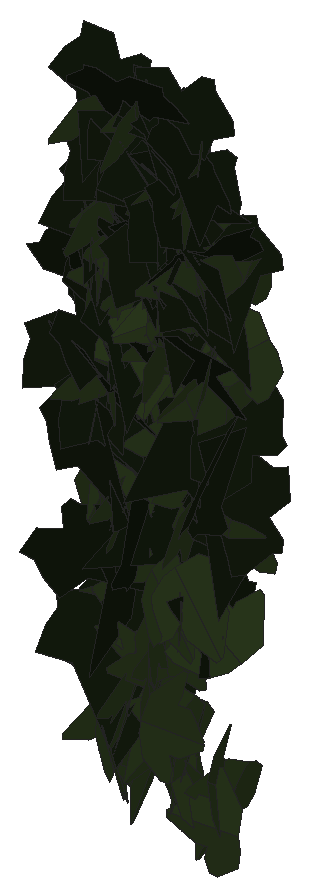
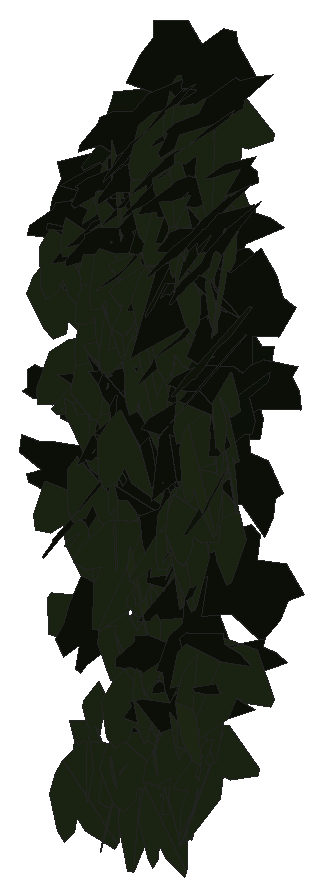
# SketchUp Ruby script. Lengths in inches.
U = 1.inch
M = Sketchup.active_model
def pt(a) = Geom::Point3d.new(a.map { |v| v * U })
def face(e, loops, mat)
  f = e.add_face(loops[0].map { |a| pt(a) })
  loops[1..].each { |l| e.add_face(l.map { |a| pt(a) }).erase! }
  f.material = f.back_material = mat if mat
  f
end
# faces: each face lists its corners as indices into pts; further lists are holes
def faces(e, pts, list, mat = nil) = list.each { |f| face(e, (f[0].is_a?(Array) ? f : [f]).map { |l| l.map { |i| pts[i] } }, mat) }
# xy, xz, yz: faces in a plane at the given z, y or x. An outline is a flat list of corners, or four numbers for a rectangle; further outlines are holes
def ring(l) = l.size == 4 ? [[l[0], l[1]], [l[2], l[1]], [l[2], l[3]], [l[0], l[3]]] : l.each_slice(2).to_a
def flat(e, list, mat, &to3) = list.each { |f| face(e, (f[0].is_a?(Array) ? f : [f]).map { |l| ring(l).map { |u, v| to3.(u, v) } }, mat) }
def xy(e, z, list, mat = nil) = flat(e, list, mat) { |x, y| [x, y, z] }
def xz(e, y, list, mat = nil) = flat(e, list, mat) { |x, z| [x, y, z] }
def yz(e, x, list, mat = nil) = flat(e, list, mat) { |y, z| [x, y, z] }
def lines(e, pts, list) = list.each { |a, b| e.add_line(pt(pts[a]), pt(pts[b])) }
# prism: a flat outline (further loops are holes) pulled along v
def prism(e, loops, v, mat = nil)
  f = face(e, loops, mat); d = Geom::Vector3d.new(v.map { |x| x * U })
  f.pushpull(f.normal.samedirection?(d) ? d.length : -d.length)
end
def box(e, o, s, mat = nil) = prism(e, [[o, [o[0] + s[0], o[1], o[2]], [o[0] + s[0], o[1] + s[1], o[2]], [o[0], o[1] + s[1], o[2]]]], [0, 0, s[2]], mat)
def at(x, y, z, deg = 0) = Geom::Transformation.translation(pt([x, y, z])) * Geom::Transformation.rotation(ORIGIN, Z_AXIS, deg.degrees)
def axes(o, x, y, z) = Geom::Transformation.new([*x, 0, *y, 0, *z, 0, *pt(o).to_a, 1])
def part(name) = M.definitions.add(name)
# library, detail: a bought-in or finely detailed component or shape, given as its bounding box
def library(name, o, s) = part(name).tap { |d| box(d.entities, o, s) }
def detail(e, o, s) = box(e.add_group.entities, o, s)
def put(e, d, t, mat = nil) = e.add_instance(d, t).tap { |i| i.material = mat if mat }
def group(e, t, mat = nil) = e.add_group.tap { |g| g.transformation = t; g.material = mat if mat }.entities
root = M.entities
M.materials.add("efeu1").color = [18, 25, 13]
M.materials.add("efeu2").color = [43, 57, 29]
c1 = part("ivyleaf_9")
p = [[1.54,2.16,1.25],[1.36,2.04,1.19],[-0.21,0.99,0.68],[-0.71,1.11,0.82],[-0.85,0.86,0.67],[-0.8,0.17,0.21],
  [-0.9,-0.01,0.1],[-0.67,-0.16,-0.02],[-0.08,-0.08,-0.05],[-0.03,-0.6,-0.4],[0.65,-0.88,-0.66],[0.83,-0.6,-0.49],
  [1.29,-0.42,-0.43],[1.8125,-0.07,-0.26],[1.21,0.44,0.15]]
faces(c1.entities,p,[[0,1,2,3,4,5,6,7,8,9,10,11,12,13,14]],"efeu1")
c2 = part("ivyleaf_10")
p = [[0,0.5,-0.03],[-0.0625,2.02,-0.43],[-0.19,2.01,-0.46],[-0.54,1.05,-0.29],[-0.52,0.625,-0.18],[-0.83,0.76,-0.28],
  [-1.16,0.64,-0.33],[-1.15,0.33,-0.24],[-0.77,-0.39,0.02],[-0.3,-0.51,0.16],[0.04,-0.48,0.23],[-0.02,2.01,-0.4375],
  [-0.06,2.01,-0.43],[0.04,-0.49,0.23],[0.67,-0.49,0.14],[1.38,0.36,-0.2],[1.375,0.51,-0.24],[0.81,0.65,-0.19],
  [0.62,0.59,-0.15],[0.6,1.09,-0.28],[0.5,1.23,-0.31]]
faces(c2.entities,p,[[0,1,2,3,4,5,6,7,8,9,10],[11,12,0,13,14,15,16,17,18,19,20]],"efeu2")
put(root,c1,axes([21.54,224.6,221.31],[-0.03751,-0.43289,0.24739],[-0.01562,-0.24695,-0.43448],[0.49835,-0.04032,0.005]))
put(root,c2,axes([21.63,224.2,216.18],[-0.33905,-0.31869,-0.18299],[0.15039,0.10685,-0.46472],[0.33531,-0.37017,0.02341]))
put(root,c2,axes([21.72,224,219.07],[0.31446,-0.36783,-0.12576],[-0.0441,0.12696,-0.4816],[0.38623,0.31398,0.0474]))
put(root,c1,axes([21.52,224,219.68],[-0.1222,-0.35359,-0.33173],[0.1348,0.30383,-0.37352],[0.46572,-0.18072,0.02107]))
put(root,c2,axes([21.77,223.86,221.06],[0.21838,-0.23586,-0.38299],[-0.07654,0.40004,-0.29001],[0.44323,0.1853,0.13862]))
put(root,c1,axes([21.34,224.08,220.3],[0.07088,-0.10152,0.48443],[0.46593,-0.15142,-0.0999],[0.16699,0.46558,0.07314]))
put(root,c2,axes([21.79,224.38,218.84],[0.0993,-0.48986,0.01339],[0.00243,-0.01317,-0.49982],[0.49003,0.09933,-0.00023]))
put(root,c2,axes([21.8,224.03,222.69],[-0.16464,-0.46488,-0.08234],[0.03056,0.07653,-0.49316],[0.47113,-0.16742,0.00321]))
put(root,c1,axes([21.51,224.42,220.18],[0.11841,-0.44827,0.18717],[0.08554,-0.1704,-0.46222],[0.47819,0.14148,0.03633]))
put(root,c1,axes([21.47,223.92,218.66],[-0.11306,-0.0302,-0.48611],[0.45319,0.17629,-0.11635],[0.17842,-0.46692,-0.01249]))
put(root,c1,axes([21.7,224.43,223],[-0.10796,-0.47713,0.10338],[-0.03629,-0.09774,-0.48901],[0.48685,-0.11309,-0.01353]))
put(root,c1,axes([21.63,224.67,221.66],[0.00983,-0.48341,0.12736],[0.02799,-0.12665,-0.48288],[0.49912,0.01662,0.02458]))
put(root,c1,axes([21.64,223.83,219.95],[0.31733,-0.28414,-0.26185],[-0.114,0.25491,-0.41476],[0.36919,0.32294,0.097]))
put(root,c2,axes([21.68,224.67,215.83],[0.13204,-0.24449,0.41568],[0.22976,-0.34703,-0.27709],[0.424,0.26419,0.02071]))
put(root,c1,axes([21.55,223.73,217.23],[-0.00624,-0.00511,-0.49993],[0.22683,0.44553,-0.00739],[0.44554,-0.22689,-0.00324]))
put(root,c2,axes([21.8125,224.49,218.18],[-0.0502,-0.33029,0.37201],[0.10917,-0.3721,-0.31564],[0.48535,0.04953,0.10947]))
put(root,c2,axes([21.9,223.93,219.46],[0.37281,-0.24376,-0.22714],[-0.08833,0.25636,-0.42009],[0.32127,0.35335,0.14809]))
put(root,c2,axes([21.625,224.31,220.9],[0.05659,-0.18533,0.46092],[0.33646,-0.32701,-0.1728],[0.3655,0.32972,0.08771]))
put(root,c2,axes([21.93,223.99,219.31],[-0.14495,-0.47492,0.05866],[-0.00922,-0.05851,-0.49648],[0.47844,-0.14501,0.0082]))
put(root,c1,axes([21.79,224.23,221.43],[-0.16768,-0.46006,-0.10113],[0.02624,0.09806,-0.48959],[0.47031,-0.1695,-0.00874]))
put(root,c1,axes([21.49,223.93,219.375],[0.3497,-0.23984,0.26493],[0.21704,-0.15194,-0.42403],[0.28391,0.41157,-0.00216]))
put(root,c2,axes([21.95,224.22,220.9],[0.07397,-0.42517,0.2525],[0.03707,-0.24982,-0.43153],[0.49311,0.08256,-0.00544]))
put(root,c1,axes([21.81,224.09,216.07],[-0.12914,-0.46255,-0.13917],[0.06065,0.12739,-0.47968],[0.47921,-0.14077,0.02321]))
put(root,c2,axes([21.96,223.97,214.81],[-0.14407,0.44926,0.16557],[-0.05725,0.15549,-0.47174],[-0.47536,-0.15489,0.00664]))
put(root,c2,axes([22.04,224.08,214.9375],[-0.31179,-0.38522,-0.06628],[0.04263,0.05077,-0.49559],[0.38855,-0.31468,0.00118]))
put(root,c1,axes([21.81,224.27,222.05],[0.02579,-0.4565,-0.20234],[0.05076,0.20396,-0.45368],[0.49675,0.00286,0.05686]))
put(root,c2,axes([22.09,224.19,221.47],[-0.22555,-0.44544,0.02654],[-0.00874,-0.02533,-0.49928],[0.44615,-0.22569,0.00364]))
put(root,c2,axes([22.05,223.81,221.57],[-0.10457,-0.43547,-0.22234],[0.04754,0.21723,-0.44783],[0.48663,-0.1148,-0.00402]))
put(root,c2,axes([22.24,224.1,215.78],[-0.41311,-0.1799,0.21673],[-0.18645,-0.11371,-0.44978],[0.21112,-0.45244,0.02686]))
put(root,c1,axes([21.92,224.44,216.65],[-0.01109,0.03453,-0.49868],[0.34864,-0.35693,-0.03247],[-0.35823,-0.34844,-0.01616]))
put(root,c1,axes([21.92,223.89,220.99],[0.3725,0.32266,0.08447],[0.06716,0.05147,-0.49279],[-0.3267,0.37847,-0.00499]))
put(root,c2,axes([22.1,224.27,217.8125],[-0.00332,-0.49995,-0.00604],[-0.00328,0.00607,-0.49995],[0.49998,-0.00328,-0.00332]))
put(root,c2,axes([21.79,223.98,217.82],[-0.2951,0.06426,-0.39848],[0.36441,-0.16984,-0.29726],[-0.17356,-0.46586,0.05341]))
put(root,c1,axes([21.89,224.03,219.14],[-0.00986,-0.35825,-0.34865],[0.03018,0.34766,-0.35808],[0.49899,-0.0281,0.01477]))
put(root,c1,axes([21.89,224.51,217.83],[-0.04094,-0.3273,0.37576],[0.07751,-0.37662,-0.31961],[0.49226,0.03209,0.08158]))
put(root,c1,axes([22.02,224.5,216.36],[-0.28969,-0.36336,-0.18453],[0.11155,0.14706,-0.46468],[0.39196,-0.3104,-0.00414]))
put(root,c2,axes([22.18,223.72,214.77],[-0.28123,0.36369,0.19656],[-0.14105,0.13906,-0.45909],[-0.3886,-0.31368,0.02438]))
put(root,c1,axes([22.07,224.48,215.63],[-0.28134,-0.40318,-0.0911],[0.05035,0.07595,-0.49163],[0.41026,-0.2858,-0.00214]))
put(root,c2,axes([22.17,224.39,222.57],[-0.16099,-0.47292,-0.02075],[0.00312,0.02086,-0.49956],[0.47336,-0.16097,-0.00376]))
put(root,c2,axes([22.27,224,220.66],[-0.32795,-0.33807,0.16781],[-0.09723,-0.13913,-0.47031],[0.36469,-0.3411,0.02551]))
put(root,c1,axes([21.93,224.38,222.47],[0.12725,-0.47335,-0.09874],[0.01766,0.10659,-0.48819],[0.48321,0.12075,0.04385]))
put(root,c2,axes([22.18,224.58,214.41],[0.10136,-0.45178,0.18875],[0.0609,-0.17962,-0.46263],[0.48582,0.11678,0.01862]))
put(root,c1,axes([22.28,223.71,223.26],[0.31921,0.28674,-0.25668],[-0.24316,-0.10821,-0.42328],[-0.2983,0.39505,0.07037]))
put(root,c2,axes([22.24,224.1,217.77],[0.11368,-0.46054,-0.15806],[-0.01495,0.15893,-0.47383],[0.48668,0.11246,0.02236]))
put(root,c2,axes([22.21,224.28,220.26],[0.02248,-0.4227,0.26612],[0.06095,-0.26208,-0.42143],[0.49576,0.05138,0.03975]))
put(root,c2,axes([22.25,224.01,215.43],[0.12561,-0.47649,0.08473],[0.03266,-0.079,-0.49264],[0.48286,0.12929,0.01128]))
put(root,c1,axes([22.22,224.21,220.71],[-0.40392,-0.1745,-0.23749],[0.22624,0.0746,-0.4396],[0.18885,-0.46259,0.01869]))
put(root,c2,axes([22.18,224.33,217.67],[-0.05004,0.49059,-0.08256],[0.01801,-0.08114,-0.49304],[-0.49716,-0.05232,-0.00956]))
put(root,c2,axes([22.3,223.96,222.75],[0.06157,-0.4591,-0.18825],[0.01634,0.19147,-0.4616],[0.49593,0.05069,0.03858]))
put(root,c1,axes([22.13,224.23,220.02],[0.01699,-0.48369,0.12551],[0.00108,-0.12555,-0.48398],[0.49971,0.01672,-0.00323]))
put(root,c2,axes([22.34,224.33,220.64],[-0.04908,-0.42906,0.25199],[0.02819,-0.2552,-0.42904],[0.49679,-0.02791,0.04924]))
put(root,c1,axes([22.07,224.22,220.99],[0.13399,-0.39431,0.2767],[0.13414,-0.2453,-0.41453],[0.46266,0.18532,0.04005]))
put(root,c2,axes([22.46,224.5625,215.73],[-0.20626,-0.36949,0.26633],[-0.02981,-0.28079,-0.41264],[0.4545,-0.1861,0.0938]))
put(root,c1,axes([22.2,224.23,222.04],[0.11358,-0.48043,-0.07928],[-0.00004,0.0814,-0.49333],[0.48693,0.11207,0.01845]))
put(root,c2,axes([22.61,224,214.92],[-0.04334,0.0762,-0.49226],[-0.19014,0.45417,0.08705],[0.4604,0.19474,-0.01039]))
put(root,c2,axes([22.58,224.5,214.92],[-0.11121,-0.35561,0.33343],[-0.08608,-0.3223,-0.37244],[0.47982,-0.14024,0.01046]))
put(root,c2,axes([22.44,224.39,215.75],[0.12072,-0.45566,0.16672],[0.07158,-0.1532,-0.47054],[0.4799,0.13748,0.02825]))
put(root,c1,axes([22.38,224.03,217.11],[0.09256,0.2493,0.42342],[-0.14507,-0.3978,0.26592],[0.46946,-0.17208,-0.00131]))
put(root,c1,axes([22.21,224.41,220.78],[0.02091,-0.31296,0.38938],[0.18516,-0.35711,-0.29696],[0.46398,0.15662,0.10096]))
put(root,c1,axes([22.3,224.6,222.65],[0.06585,-0.48486,0.10284],[0.00673,-0.10286,-0.48926],[0.4956,0.06582,-0.00702]))
put(root,c1,axes([22.36,224.57,222.28],[-0.02633,-0.49762,0.04098],[-0.01268,-0.04036,-0.49821],[0.49915,-0.02728,-0.0105]))
put(root,c2,axes([22.57,224.22,221.76],[0.08333,-0.45133,0.19838],[0.02595,-0.1969,-0.45886],[0.49232,0.08677,-0.00939]))
put(root,c2,axes([22.59,224.32,219.61],[0.08317,-0.49286,0.01312],[0.0011,-0.01312,-0.49983],[0.49303,0.08317,-0.0011]))
put(root,c1,axes([22.21,224.35,221.67],[0.22292,-0.30335,0.32907],[0.19664,-0.26386,-0.37644],[0.40204,0.29725,0.00167]))
put(root,c1,axes([22.88,223.66,221.05],[-0.03501,0.07217,0.49352],[-0.24708,0.42726,-0.08001],[-0.43327,-0.24949,0.00575]))
put(root,c1,axes([22.25,223.9,221.87],[0.12975,0.09374,-0.47369],[0.25659,0.40212,0.14986],[0.40906,-0.28198,0.05624]))
put(root,c2,axes([22.74,224.23,214.4],[-0.46927,0.12236,0.12173],[-0.11844,0.02824,-0.48495],[-0.12555,-0.48397,0.00248]))
put(root,c1,axes([22.5,224.57,222.8],[-0.08465,-0.48673,-0.07697],[0.00685,0.07693,-0.494],[0.49273,-0.08469,-0.00635]))
put(root,c2,axes([22.66,224.13,215.75],[-0.3068,-0.37979,-0.10783],[-0.06748,-0.08411,0.48823],[-0.389,0.31414,0.00035]))
put(root,c2,axes([22.53,223.91,220.07],[0.47802,0.14225,0.03556],[0.03133,0.01937,-0.49864],[-0.14324,0.47895,0.00961]))
put(root,c2,axes([22.74,224.25,219.99],[-0.14689,-0.47623,0.04032],[-0.01078,-0.03887,-0.49837],[0.47781,-0.14729,0.00116]))
put(root,c1,axes([22.57,224.2,222.12],[-0.09462,-0.48912,-0.04255],[0.00434,0.0425,-0.49817],[0.49095,-0.09464,-0.0038]))
put(root,c2,axes([22.83,223.77,216.42],[-0.09102,0.37385,0.3193],[-0.24065,0.24929,-0.36047],[-0.42872,-0.2193,0.13455]))
put(root,c2,axes([22.71,224.03,220.35],[-0.06826,0.38315,0.3139],[-0.05596,0.30887,-0.38919],[-0.49215,-0.08826,0.00071]))
put(root,c2,axes([22.78,224.27,218.66],[-0.16791,-0.42312,0.20683],[0.01084,-0.22299,-0.44739],[0.47084,-0.14576,0.08405]))
put(root,c2,axes([22.92,224.34,220.34],[-0.13915,-0.00961,0.48015],[-0.17355,-0.46511,-0.05961],[0.44779,-0.18324,0.12611]))
put(root,c2,axes([22.97,223.95,216.86],[-0.20618,0.33232,0.31154],[-0.33485,0.12126,-0.35096],[-0.30881,-0.35336,0.17255]))
put(root,c1,axes([23.03,224.17,217.78],[-0.0048,-0.01789,-0.49966],[-0.20907,-0.45382,0.01826],[-0.45416,0.20911,-0.00312]))
put(root,c1,axes([22.73,224.65,222.06],[-0.14997,-0.45868,0.13087],[-0.02432,-0.12965,-0.48229],[0.47636,-0.15102,0.01658]))
put(root,c2,axes([22.76,224.23,217.23],[-0.35048,-0.30604,-0.18304],[0.16378,0.08984,-0.4638],[0.31676,-0.38506,0.03727]))
put(root,c1,axes([22.73,224.1,218.29],[-0.3371,0.1887,0.31742],[0.2772,-0.15466,0.38632],[0.24398,0.43643,-0.00034]))
put(root,c1,axes([22.73,224.52,221.27],[-0.10668,-0.48417,-0.06479],[0.0154,0.06295,-0.49578],[0.48824,-0.10777,0.00148]))
put(root,c2,axes([22.5625,224.42,215.85],[-0.27637,0.02431,0.41596],[0.41554,-0.02076,0.2773],[0.03075,0.49898,-0.00872]))
put(root,c2,axes([22.9,224.34,220.71],[-0.03192,-0.49498,-0.06309],[0.00247,0.06306,-0.496],[0.49897,-0.03197,-0.00158]))
put(root,c2,axes([22.78,224.45,214.85],[0.13996,-0.31109,0.36556],[0.21039,-0.3025,-0.33798],[0.43145,0.24842,0.04623]))
put(root,c2,axes([22.93,223.73,220.12],[-0.02939,-0.28178,-0.41199],[0.04683,0.40933,-0.2833],[0.49693,-0.05524,0.00233]))
put(root,c2,axes([23.09,224.11,214.01],[-0.05633,0.35643,-0.3461],[-0.14609,0.32103,0.35439],[0.47485,0.14105,0.06797]))
put(root,c2,axes([22.98,224.24,220.89],[-0.13532,-0.47539,-0.07543],[0.00977,0.07563,-0.49415],[0.48124,-0.13521,-0.01118]))
put(root,c1,axes([22.73,223.98,221.65],[0.17773,-0.45374,-0.11194],[-0.01877,0.11273,-0.48676],[0.46697,0.17722,0.02303]))
put(root,c2,axes([22.97,224.21,222.08],[0.16141,-0.45303,-0.13677],[0.00389,0.14577,-0.47826],[0.47321,0.15333,0.05058]))
put(root,c2,axes([23.01,223.5,215.33],[-0.08171,0.27456,0.40981],[-0.10727,0.39556,-0.2864],[-0.48147,-0.13473,-0.00574]))
put(root,c1,axes([22.83,224.3,220.65],[-0.01909,-0.47642,0.15053],[0.02018,-0.15125,-0.47615],[0.49923,-0.0121,0.025]))
put(root,c2,axes([23.05,224.23,220.375],[-0.13063,-0.47526,-0.08406],[0.01358,0.08343,-0.4928],[0.48244,-0.13103,-0.00889]))
put(root,c2,axes([22.97,223.66,217.02],[-0.05345,0.47416,0.14939],[-0.0107,0.14912,-0.47712],[-0.49702,-0.0542,-0.0058]))
put(root,c1,axes([22.77,223.76,221.44],[-0.00455,-0.29501,-0.40367],[0.16377,0.38053,-0.27995],[0.4724,-0.13476,0.09317]))
put(root,c2,axes([23.02,224.22,221.64],[0.03335,-0.41032,0.28376],[0.07722,-0.27673,-0.40922],[0.49287,0.07112,0.04491]))
put(root,c2,axes([23.14,224.33,218.13],[-0.14998,-0.45529,0.14218],[-0.02968,-0.13984,-0.47913],[0.47605,-0.15215,0.01492]))
put(root,c2,axes([22.8,224.19,219.38],[-0.22493,-0.1948,-0.40182],[0.39253,0.12825,-0.2819],[0.21289,-0.44227,0.09523]))
put(root,c2,axes([23.08,224.02,217.92],[0.1073,-0.4532,-0.18192],[0.01232,0.18872,-0.46285],[0.4882,0.09484,0.05167]))
put(root,c1,axes([23.01,224.28,218.74],[0.11813,-0.19734,-0.44396],[0.20107,-0.39607,0.22956],[-0.44229,-0.23277,-0.01422]))
put(root,c2,axes([23.16,224.51,219.5],[-0.04549,0.13802,-0.47842],[-0.17851,-0.45299,-0.11371],[-0.46483,0.16046,0.09049]))
put(root,c1,axes([22.92,223.73,220.02],[0.48212,0.13236,0.00633],[0.00608,0.00174,-0.49996],[-0.13237,0.48216,0.00007]))
put(root,c1,axes([23.13,224.68,216.15],[-0.00798,0.03231,0.49889],[-0.23532,-0.44047,0.02476],[0.44109,-0.2344,0.02224]))
put(root,c1,axes([22.9,224.25,222.3],[0.05525,-0.40646,0.2859],[0.13276,-0.26513,-0.40259],[0.47887,0.1204,0.07863]))
put(root,c2,axes([23.12,224.07,221.64],[-0.11664,0.48116,-0.06987],[0.01797,-0.06754,-0.49509],[-0.48587,-0.11801,-0.00154]))
put(root,c2,axes([23.31,224.36,216.1],[0.21951,0.36568,0.26095],[-0.14332,-0.21826,0.42641],[0.42577,-0.262,0.009]))
put(root,c1,axes([22.97,223.91,221.9],[0.28791,-0.40413,-0.06157],[-0.02794,0.05567,-0.4961],[0.40783,0.28911,0.00947]))
put(root,c2,axes([23.28,224.18,221.16],[-0.167,-0.47127,0.00322],[-0.00102,-0.00305,-0.49999],[0.47128,-0.16701,0.00005]))
put(root,c1,axes([23.37,223.9,221.36],[0.02504,0.47073,-0.1667],[-0.02984,-0.1652,-0.47098],[-0.49848,0.03354,0.01982]))
put(root,c2,axes([23.32,223.85,221.12],[-0.26532,-0.4229,0.02762],[-0.01577,-0.02271,-0.49923],[0.4235,-0.26579,-0.00128]))
put(root,c1,axes([23.03,224.01,218.05],[-0.17077,0.18079,0.43377],[0.298,-0.3152,0.24869],[0.36337,0.34346,-0.0001]))
put(root,c2,axes([23.36,224,220.03],[0.20904,-0.3634,-0.27247],[-0.09174,0.25998,-0.41713],[0.44484,0.22438,0.04202]))
put(root,c2,axes([23.32,224.53,214.31],[-0.02268,-0.44254,0.23161],[0.00189,-0.23193,-0.44295],[0.49948,-0.01922,0.01219]))
put(root,c2,axes([23.16,223.82,217.03],[0.176,0.42272,0.20082],[0.04346,0.19886,-0.45669],[-0.46598,0.17821,0.03326]))
put(root,c2,axes([23.35,224.35,219.34],[-0.29105,-0.40627,0.01545],[-0.00919,-0.01242,-0.49976],[0.40646,-0.29119,-0.00024]))
put(root,c1,axes([23.17,224.46,221.27],[-0.19886,-0.39924,-0.22596],[0.10338,0.20094,-0.44602],[0.44695,-0.22411,0.00262]))
put(root,c2,axes([23.46,224.28,217.64],[-0.47192,-0.09404,0.13582],[-0.13021,-0.04125,-0.48098],[0.10167,-0.48934,0.01444]))
put(root,c1,axes([23.64,224.35,218.74],[-0.4488,-0.18932,-0.11287],[-0.09574,-0.06319,0.48666],[-0.19853,0.45844,0.02047]))
put(root,c1,axes([23.16,224.12,220.98],[0.09704,-0.42696,-0.24143],[-0.02467,0.24155,-0.43709],[0.48987,0.09674,0.02581]))
put(root,c1,axes([23.21,224.63,217.68],[0.03036,-0.45351,0.20835],[0.00203,-0.20862,-0.45439],[0.49907,0.02843,-0.01083]))
put(root,c1,axes([23.79,224.45,217.89],[-0.37082,0.05543,0.33079],[-0.32589,0.05703,-0.37489],[-0.07929,-0.49363,-0.00616]))
put(root,c2,axes([23.77,223.8,214.11],[-0.04619,0.11027,0.4855],[-0.49784,-0.01446,-0.04408],[0.00432,-0.48748,0.11113]))
put(root,c1,axes([23.24,223.84,218.14],[-0.04078,0.39959,0.29777],[0.03205,-0.29605,0.40166],[0.4973,0.05185,-0.00147]))
put(root,c2,axes([23.6,223.82,214.65],[-0.11469,0.2255,0.43127],[-0.30883,0.30872,-0.24355],[-0.37612,-0.32225,0.06847]))
put(root,c2,axes([23.46,224.47,220.84],[-0.0959,-0.46905,0.14422],[0.00544,-0.14795,-0.47758],[0.49069,-0.09003,0.03348]))
put(root,c2,axes([23.75,224.34,220.11],[-0.30253,0.05444,0.39435],[-0.3759,-0.20212,-0.26047],[0.13105,-0.45408,0.16322]))
